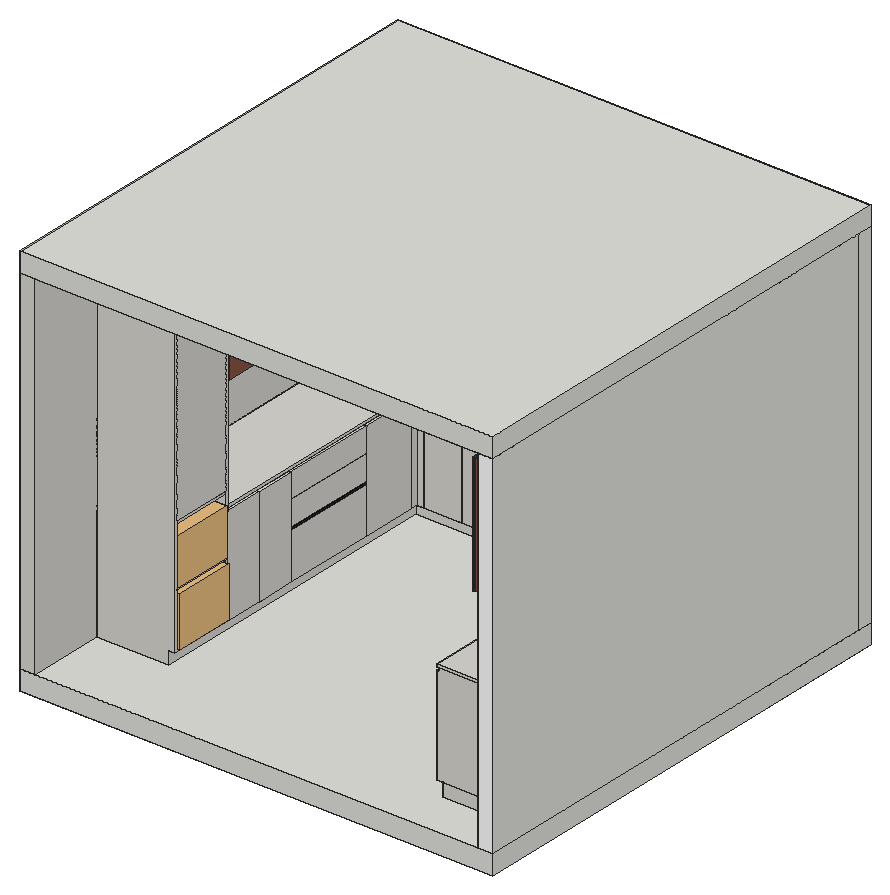
# SketchUp Ruby script. Lengths in inches.
U = 1.inch
M = Sketchup.active_model
def pt(a) = Geom::Point3d.new(a.map { |v| v * U })
def face(e, loops, mat)
  f = e.add_face(loops[0].map { |a| pt(a) })
  loops[1..].each { |l| e.add_face(l.map { |a| pt(a) }).erase! }
  f.material = f.back_material = mat if mat
  f
end
# faces: each face lists its corners as indices into pts; further lists are holes
def faces(e, pts, list, mat = nil) = list.each { |f| face(e, (f[0].is_a?(Array) ? f : [f]).map { |l| l.map { |i| pts[i] } }, mat) }
# xy, xz, yz: faces in a plane at the given z, y or x. An outline is a flat list of corners, or four numbers for a rectangle; further outlines are holes
def ring(l) = l.size == 4 ? [[l[0], l[1]], [l[2], l[1]], [l[2], l[3]], [l[0], l[3]]] : l.each_slice(2).to_a
def flat(e, list, mat, &to3) = list.each { |f| face(e, (f[0].is_a?(Array) ? f : [f]).map { |l| ring(l).map { |u, v| to3.(u, v) } }, mat) }
def xy(e, z, list, mat = nil) = flat(e, list, mat) { |x, y| [x, y, z] }
def xz(e, y, list, mat = nil) = flat(e, list, mat) { |x, z| [x, y, z] }
def yz(e, x, list, mat = nil) = flat(e, list, mat) { |y, z| [x, y, z] }
def lines(e, pts, list) = list.each { |a, b| e.add_line(pt(pts[a]), pt(pts[b])) }
# prism: a flat outline (further loops are holes) pulled along v
def prism(e, loops, v, mat = nil)
  f = face(e, loops, mat); d = Geom::Vector3d.new(v.map { |x| x * U })
  f.pushpull(f.normal.samedirection?(d) ? d.length : -d.length)
end
def box(e, o, s, mat = nil) = prism(e, [[o, [o[0] + s[0], o[1], o[2]], [o[0] + s[0], o[1] + s[1], o[2]], [o[0], o[1] + s[1], o[2]]]], [0, 0, s[2]], mat)
def at(x, y, z, deg = 0) = Geom::Transformation.translation(pt([x, y, z])) * Geom::Transformation.rotation(ORIGIN, Z_AXIS, deg.degrees)
def axes(o, x, y, z) = Geom::Transformation.new([*x, 0, *y, 0, *z, 0, *pt(o).to_a, 1])
def part(name) = M.definitions.add(name)
# library, detail: a bought-in or finely detailed component or shape, given as its bounding box
def library(name, o, s) = part(name).tap { |d| box(d.entities, o, s) }
def detail(e, o, s) = box(e.add_group.entities, o, s)
def put(e, d, t, mat = nil) = e.add_instance(d, t).tap { |i| i.material = mat if mat }
def group(e, t, mat = nil) = e.add_group.tap { |g| g.transformation = t; g.material = mat if mat }.entities
root = M.entities
M.materials.add("Pionite-a-Panolam-Brand-Canyon-Shadow-SO200-4K").color = [135, 86, 67]
M.materials.add("Tafisa-Cachemire-or-Cashmere-PM776-4K").color = [217, 215, 209]
M.materials.add("[Color M00]").color = [255, 255, 255]
M.materials.add("[Color M09]").color = [0, 0, 0]
M.materials.add("[Translucent Glass Gray]").color = [128, 128, 128]
M.materials["[Translucent Glass Gray]"].alpha = 0.5
c1 = library("Bowl 296 012 003",[-3.97,-3.98,-0.03],[7.96,7.96,3.84])
c2 = library("Cooker 143 035",[-7,-5.69,0],[14,11.41,9.46])
c3 = library("Cup 287 006 002",[-2.07,-2.07,-0.01],[4.14,4.15,3.07])
c4 = library("Kitchen Props 134 014",[-15.6875,-7.04,0],[31.37,14.09,12.97])
c5 = library("2-FOUR H60 CLC2",[0,-1.47,0],[23.5,21.86,23.5])
c6 = library("2-MICRO H40 CLC2",[0,-1.47,0],[23.5,21.86,15.63])
c7 = library("Stand 298 006",[-6.74,-6.74,-0.04],[13.48,13.48,13.7])
c8 = library("Bowl 298 014 002",[-6.91,-6.91,-0.04],[13.82,13.82,6.19])
c9 = library("Jug 155 004",[-2.86,-2.52,0],[7.11,5.04,4.97])
c10 = library("Jar 134 013",[-1.97,-1.98,0],[3.94,3.95,4.83])
c11 = library("Candle 160 011",[-1.94,-2,0],[3.88,3.94,4.57])
c12 = library("Jar 83-03",[-2.15,-2.09,0],[4.3,4.18,5.88])
c13 = library("5-HOTTE ASPIRANTE CLC2",[-15.16,-17.72,-0.29],[30.34,17.72,30.09])
c14 = library("Wicker-wood basket",[2.36,-2.2,-7.41],[20.73,22.5,7.78])
c15 = part("Group\#13")
box(c15.entities,[0,0,-0.71],[22.83,18.58,0.71])
c16 = library("Группа\#68",[0,0,-0.08],[23.6,20.47,1.99])
c17 = part("Group\#31")
xy(c17.entities,0,[[0.93,0,0.71,0.01,0.49,0.07,0.31,0.1875,0.16,0.35,0.05,0.54,0,0.76,0.01,0.98,0.07,1.1875,0.1875,1.375,0.35,1.53,0.54,1.63,0.76,1.68,0.98,1.68,1.1875,1.61,1.375,1.5,1.53,1.33,1.63,1.14,1.68,0.93,1.68,0.71,1.61,0.49,1.5,0.31,1.33,0.16,1.14,0.05]])
xz(root,126.85,[[20.33,66.28,37.04,101.29],[107.08,66.28,123.67,101.29]],"[Translucent Glass Gray]")
yz(root,17.15,[[107.09,66.28,123.67,101.29]],"[Translucent Glass Gray]")
yz(root,126.85,[[107.375,66.28,123.67,101.29]],"[Translucent Glass Gray]")
put(root,c1,at(32.52,133.57,66.28))
put(root,c1,at(24.37,133.35,66.28))
put(root,c2,at(33.29,126.21,41.57))
put(root,c3,at(32.73,133.83,78.66))
put(root,c3,at(28.04,133.83,78.66))
put(root,c3,at(23.35,133.83,78.66))
put(root,c4,axes([122.51,100.875,41.57],[-1,0,0],[0,1,0],[0,0,1]))
put(root,c5,axes([28.46,24.09,11.01],[0,0.79062,0],[-0.71131,0,0],[0,0,0.64648]))
put(root,c6,axes([28,24.09,27.71],[0,0.79062,0],[-0.6156,0,0],[0,0,0.91109]))
put(root,c7,axes([120.65,133.01,66.3],[0.3355,0,0],[0,0.3355,0],[0,0,0.3355]))
put(root,c7,axes([115.03,133.01,66.3],[0.3355,0,0],[0,0.3355,0],[0,0,0.3355]))
put(root,c7,axes([109.78,133.01,66.3],[0.3355,0,0],[0,0.3355,0],[0,0,0.3355]))
put(root,c8,axes([34.09,132.09,90.3],[0.31894,0,0],[0,0.31894,0],[0,0,0.31894]))
put(root,c8,axes([28.66,132.09,90.3],[0.31894,0,0],[0,0.31894,0],[0,0,0.31894]))
put(root,c8,axes([23.47,132.09,90.3],[0.31894,0,0],[0,0.31894,0],[0,0,0.31894]))
put(root,c9,axes([120.81,133.09,78.66],[0.59397,0.59397,0],[-0.59397,0.59397,0],[0,0,0.84]))
put(root,c9,axes([115.38,133.09,78.66],[0.59397,0.59397,0],[-0.59397,0.59397,0],[0,0,0.84]))
put(root,c9,axes([109.94,133.09,78.66],[0.59397,0.59397,0],[-0.59397,0.59397,0],[0,0,0.84]))
put(root,c10,at(120.52,132.59,90.33))
put(root,c11,axes([16.52,127.52,41.57],[1.7,0,0],[0,1.7,0],[0,0,1.7]))
put(root,c12,at(115,132.73,90.33))
put(root,c12,at(109.8,132.73,90.33))
put(root,c13,axes([72.24,139.5,63.27],[0.99919,0,0],[0,1,0],[0,0,1]))
g1 = group(root,at(0,0,0))
box(g1,[0,0,0],[144,144,6])
g2 = group(root,at(0,139.5,6))
xy(g2,0,[[0,0,144,4.5]])
xy(g2,108,[[0,0,144,4.5]])
xz(g2,0,[[[0,0,144,108],[4.5,35.57,139.5,59.57]],[4.5,35.57,139.5,59.57]])
xz(g2,4.5,[[0,0,144,108]])
yz(g2,0,[[0,0,4.5,108]])
yz(g2,144,[[0,0,4.5,108]])
g3 = group(root,at(139.5,0,6))
xy(g3,0,[[0,0,4.5,139.5]])
xy(g3,108,[[0,0,4.5,139.5]],"[Color M00]")
xz(g3,0,[[0,0,4.5,108]],"[Color M00]")
xz(g3,139.5,[[0,0,4.5,108]])
yz(g3,0,[[0,0,0,108,139.5,108,139.5,59.57,14.26,59.57,14.26,35.57,139.5,35.57,139.5,0],[14.26,35.57,139.5,59.57]])
yz(g3,4.5,[[0,0,139.5,108]])
g4 = group(root,at(0,0,6),"Tafisa-Cachemire-or-Cashmere-PM776-4K")
xy(g4,0,[[0,0,4.5,139.5]])
xy(g4,108,[[0,0,4.5,139.5]])
xz(g4,0,[[0,0,4.5,108]])
xz(g4,139.5,[[0,0,4.5,108]])
yz(g4,0,[[0,0,139.5,108]])
yz(g4,4.5,[[0,0,139.5,0,139.5,35.57,43.38,35.57,43.38,59.57,139.5,59.57,139.5,108,0,108],[43.38,35.57,139.5,59.57]])
g5 = group(root,at(4.5,0,6),"Tafisa-Cachemire-or-Cashmere-PM776-4K")
xy(g5,0,[[113,14.26,113,117.5,22,117.5,22,23.38,0,23.38,0,139.5,135,139.5,135,14.26]])
xy(g5,4,[[111,14.26,111,38.26,111.71,38.26,111.71,38.38,111,38.38,111,50.26,111.71,50.26,111.71,50.38,111,50.38,111,62.26,111.71,62.26,111.71,62.38,111,62.38,111,72.38,111.71,72.38,111.71,72.5,111,72.5,111,99.38,111.71,99.38,111.71,99.5,111,99.5,111,113.38,111.71,113.38,111.71,113.5,111,113.5,111,115.5,113,115.5,113,14.26],[22,23.38,22,115.5,24,115.5,24,113.5,23.29,113.5,23.29,113.38,24,113.38,24,96.5,23.29,96.5,23.29,96.38,24,96.38,24,67.62,23.29,67.62,23.29,67.5,24,67.5,24,55.5,23.29,55.5,23.29,55.38,24,55.38,24,43.5,23.29,43.5,23.29,43.38,24,43.38,24,23.38],[22,115.5,22,117.5,113,117.5,113,115.5,109.12,115.5,109.12,116.21,109,116.21,109,115.5,97.37,115.5,97.37,116.21,97.25,116.21,97.25,115.5,85.5,115.5,85.5,116.21,85.38,116.21,85.38,115.5,49.62,115.5,49.62,116.21,26,116.21,26,115.5],[26.12,115.5,37.75,116.21],[37.87,115.5,49.5,116.21]])
xy(g5,4.71,[[111,14.97,133.83,37.56],[1.17,24.09,24,42.67]])
xy(g5,18.02,[[111,72.5,111.71,99.38]])
xy(g5,18.02,[[23.29,67.62,24,96.38],[49.62,115.5,85.38,116.21]],"[Color M09]")
xy(g5,19,[[111,72.5,111.71,99.38]])
xy(g5,19,[[23.29,67.62,24,96.38],[49.62,115.5,85.38,116.21]],"[Color M09]")
xy(g5,26.5,[[23.29,67.62,24,96.38],[111,72.5,111.71,99.38],[49.62,115.5,85.38,116.21]])
xy(g5,26.62,[[23.29,67.62,24,96.38],[111,72.5,111.71,99.38],[49.62,115.5,85.38,116.21]])
xy(g5,33.29,[[111,14.97,133.83,37.56]])
xy(g5,34,[[111,14.26,111.71,38.26],[111,38.38,111.71,50.26],[23.29,43.5,24,55.38],[111,50.38,111.71,62.26],[23.29,55.5,24,67.5],
  [111,62.38,111.71,72.38],[23.29,67.62,24,96.38],[111,72.5,111.71,99.38],[23.29,96.5,24,113.38],[111,99.5,111.71,113.38],
  [23.29,113.5,24,115.5],[111,113.5,111.71,115.5],[23.29,115.5,26,116.21],[26.12,115.5,37.75,116.21],[37.87,115.5,49.5,116.21],
  [49.62,115.5,85.38,116.21],[85.5,115.5,97.25,116.21],[97.37,115.5,109,116.21],[109.12,115.5,111.71,116.21]])
xy(g5,34.79,[[111,14.26,111.71,115.5],[23.29,43.5,24,115.5],[23.29,115.5,111.71,116.21]])
xy(g5,35.57,[[111,14.26,135,14.26,135,139.5,0,139.5,0,43.38,23.29,43.38,23.29,43.5,24,43.5,24,115.5,111,115.5]])
xy(g5,39.83,[[1.17,24.09,1.17,42.67,23.29,42.67,23.29,42.56,24,42.56,24,24.21,23.29,24.21,23.29,24.09]])
xy(g5,107.17,[[23.29,24.21,24,42.56]])
xy(g5,107.29,[[1.17,24.09,23.29,42.67],[23.29,24.09,24,24.21],[23.29,24.21,24,42.56],[23.29,42.56,24,42.67]])
xy(g5,108,[[0,23.38,24,43.38]])
xz(g5,14.26,[[113,0,135,4],[111,4,135,4,135,34.79,111.71,34.79,111.71,34,111,34],[111,34.79,135,35.57]])
xz(g5,14.97,[[111,4.71,133.83,33.29]])
xz(g5,23.38,[[0,0,22,0,22,4,24,4,24,108,0,108]])
xz(g5,24.09,[[1.17,4.71,24,39.83],[1.17,39.83,23.29,107.29],[23.29,39.83,24,107.29]])
xz(g5,24.21,[[23.29,39.83,24,107.17]])
xz(g5,37.56,[[111,4.71,133.83,33.29]])
xz(g5,38.26,[[111,4,111.71,34]])
xz(g5,38.38,[[111,4,111.71,34]])
xz(g5,42.56,[[23.29,39.83,24,107.17]])
xz(g5,42.67,[[1.17,4.71,24,39.83],[1.17,39.83,23.29,107.29],[23.29,39.83,24,107.29]])
xz(g5,43.38,[[23.29,4,24,34],[23.29,34,24,34.79],[23.29,34.79,24,108],[0,35.57,23.29,108]])
xz(g5,43.5,[[23.29,4,24,34],[23.29,34.79,24,35.57]])
xz(g5,50.26,[[111,4,111.71,34]])
xz(g5,50.38,[[111,4,111.71,34]])
xz(g5,55.38,[[23.29,4,24,34]])
xz(g5,55.5,[[23.29,4,24,34]])
xz(g5,62.26,[[111,4,111.71,34]])
xz(g5,62.38,[[111,4,111.71,34]])
xz(g5,67.5,[[23.29,4,24,18.02],[23.29,18.02,24,19],[23.29,19,24,26.5],[23.29,26.5,24,26.62],[23.29,26.62,24,34]])
xz(g5,67.62,[[23.29,4,24,18.02],[23.29,19,24,26.5],[23.29,26.62,24,34]])
xz(g5,72.38,[[111,4,111.71,18.02],[111,18.02,111.71,19],[111,19,111.71,26.5],[111,26.5,111.71,26.62],[111,26.62,111.71,34]])
xz(g5,72.5,[[111,4,111.71,18.02],[111,19,111.71,26.5],[111,26.62,111.71,34]])
xz(g5,96.38,[[23.29,4,24,18.02],[23.29,19,24,26.5],[23.29,26.62,24,34]])
xz(g5,96.5,[[23.29,4,24,18.02],[23.29,18.02,24,19],[23.29,19,24,26.5],[23.29,26.5,24,26.62],[23.29,26.62,24,34]])
xz(g5,99.38,[[111,4,111.71,18.02],[111,19,111.71,26.5],[111,26.62,111.71,34]])
xz(g5,99.5,[[111,4,111.71,34]])
xz(g5,113.38,[[23.29,4,24,34],[111,4,111.71,34]])
xz(g5,113.5,[[23.29,4,24,34],[111,4,111.71,34]])
xz(g5,115.5,[[24,4,26,34],[26.12,4,37.75,34],[37.87,4,49.5,34],[49.62,4,85.38,18.02],[85.5,4,97.25,34],
  [97.37,4,109,34],[109.12,4,111,34],[49.62,19,85.38,26.5],[49.62,26.62,85.38,34],[24,34.79,111,35.57]])
xz(g5,116.21,[[26,4,26.12,34],[26.12,4,37.75,34],[37.75,4,37.87,34],[37.87,4,49.5,34],[49.5,4,49.62,18.02],
  [85.38,4,85.5,18.02],[97.25,4,97.37,34],[109,4,109.12,34],[49.5,19,49.62,26.5],[85.38,19,85.5,26.5],
  [49.5,26.5,85.5,26.62],[49.5,26.62,49.62,34],[85.38,26.62,85.5,34]])
xz(g5,116.21,[[49.5,18.02,85.5,19],[23.29,34,111.71,34.79]],"[Color M09]")
xz(g5,117.5,[[22,0,113,4]])
xz(g5,139.5,[[0,0,135,34],[0,34,135,34.79],[0,34.79,135,35.57]])
yz(g5,0,[[23.38,0,139.5,34],[23.38,34,139.5,34.79],[23.38,34.79,23.38,108,43.38,108,43.38,35.57,139.5,35.57,139.5,34.79]])
yz(g5,1.17,[[24.09,4.71,42.67,39.83],[24.09,39.83,42.67,107.29]])
yz(g5,22,[[23.38,0,117.5,4]])
yz(g5,23.29,[[43.38,4,43.5,34],[55.38,4,55.5,34],[67.5,4,67.62,18.02],[96.38,4,96.5,18.02],[113.38,4,113.5,34],
  [67.5,19,67.62,26.5],[96.38,19,96.5,26.5],[67.5,26.5,96.5,26.62],[67.5,26.62,67.62,34],[96.38,26.62,96.5,34],
  [43.38,34.79,43.5,35.57],[24.09,39.83,24.21,107.29],[42.56,39.83,42.67,107.29],[24.21,107.17,42.56,107.29]])
yz(g5,23.29,[[67.5,18.02,96.5,19],[43.38,34,116.21,34.79]],"[Color M09]")
yz(g5,24,[[[23.38,4,43.38,108],[24.09,4.71,42.67,107.29]],[43.5,4,55.38,34],[55.5,4,67.5,34],[67.62,4,96.38,18.02],[96.5,4,113.38,34],
  [113.5,4,115.5,34],[67.62,19,96.38,26.5],[67.62,26.62,96.38,34],[43.5,34.79,115.5,35.57],[24.21,39.83,42.56,107.17]])
yz(g5,26,[[115.5,4,116.21,34]])
yz(g5,26.12,[[115.5,4,116.21,34]])
yz(g5,37.75,[[115.5,4,116.21,34]])
yz(g5,37.87,[[115.5,4,116.21,34]])
yz(g5,49.5,[[115.5,4,116.21,18.02],[115.5,18.02,116.21,19],[115.5,19,116.21,26.5],[115.5,26.5,116.21,26.62],[115.5,26.62,116.21,34]])
yz(g5,49.62,[[115.5,4,116.21,18.02],[115.5,19,116.21,26.5],[115.5,26.62,116.21,34]])
yz(g5,85.38,[[115.5,4,116.21,18.02],[115.5,19,116.21,26.5],[115.5,26.62,116.21,34]])
yz(g5,85.5,[[115.5,4,116.21,18.02],[115.5,18.02,116.21,19],[115.5,19,116.21,26.5],[115.5,26.5,116.21,26.62],[115.5,26.62,116.21,34]])
yz(g5,97.25,[[115.5,4,116.21,34]])
yz(g5,97.37,[[115.5,4,116.21,34]])
yz(g5,109,[[115.5,4,116.21,34]])
yz(g5,109.12,[[115.5,4,116.21,34]])
yz(g5,111,[[[14.26,4,38.26,34],[14.97,4.71,37.56,33.29]],[38.38,4,50.26,34],[50.38,4,62.26,34],[62.38,4,72.38,34],[72.5,4,99.38,18.02],
  [99.5,4,113.38,34],[113.5,4,115.5,34],[72.5,19,99.38,26.5],[72.5,26.62,99.38,34],[14.26,34.79,115.5,35.57]])
yz(g5,111.71,[[38.26,4,38.38,34],[50.26,4,50.38,34],[62.26,4,62.38,34],[72.38,4,72.5,18.02],[99.38,4,99.5,34],
  [113.38,4,113.5,34],[72.38,19,72.5,26.5],[72.38,26.5,99.38,26.62],[72.38,26.62,72.5,34]])
yz(g5,111.71,[[72.38,18.02,99.38,19],[14.26,34,116.21,34.79]],"[Color M09]")
yz(g5,113,[[14.26,0,117.5,4]])
yz(g5,133.83,[[14.97,4.71,37.56,33.29]])
yz(g5,135,[[14.26,0,139.5,34],[14.26,34,139.5,34.79],[14.26,34.79,139.5,35.57]])
put(g5,c14,at(109,17.26,12.81))
put(g5,c14,at(109,17.26,22.11))
put(g5,c14,at(108.64,17.26,31.4))
put(g5,c15,at(1.17,24.09,21.71))
put(g5,c15,at(1.17,24.09,39.71))
g6 = group(root,at(4.5,43.38,65.57),"Pionite-a-Panolam-Brand-Canyon-Shadow-SO200-4K")
xy(g6,0,[[122.71,-29.12,122.71,81.12,122,81.12,122,83.12,120,83.12,120,83.83,15,83.83,15,83.12,13,83.12,13,81.12,12.29,81.12,12.29,0,0,0,0,96.12,135,96.12,135,-29.12],[122,-29.12,122.71,-7.83],[122,-7.72,122.71,10.17],[12.29,0,13,14.38],[122,10.28,122.71,28.17],
  [12.29,14.5,13,28.88],[122,28.28,122.71,46.17],[12.29,29,13,45.88],[12.29,46,13,62.88],[122,46.28,122.71,63.17],
  [122,63.28,122.71,81],[33.37,83.12,51.5,83.83],[51.62,83.12,67.5,83.83],[67.62,83.12,83.5,83.83],[83.62,83.12,101.75,83.83]])
xy(g6,0,[[12.29,63,13,81],[15.12,83.12,33.25,83.83],[101.87,83.12,119.88,83.83]],"[Color M09]")
xy(g6,0.71,[[1,63.71,12.29,80.29],[122.71,63.99,134,80.29],[15.83,83.83,32.54,95.12],[102.58,83.83,119.17,95.12]])
xy(g6,0.71,[[12.29,63.71,13,80.29],[122,63.99,122.71,80.29],[15.83,83.12,32.54,83.83],[102.58,83.12,119.17,83.83]],"[Color M09]")
xy(g6,35.72,[[1,63.71,12.29,80.29],[122.71,63.99,134,80.29],[15.83,83.83,32.54,95.12],[102.58,83.83,119.17,95.12]])
xy(g6,35.72,[[12.29,63.71,13,80.29],[122,63.99,122.71,80.29],[15.83,83.12,32.54,83.83],[102.58,83.12,119.17,83.83]],"[Color M09]")
xy(g6,36.43,[[122.71,-29.12,135,-29.12,135,96.12,0,96.12,0,0,12.29,0,12.29,81.12,13,81.12,13,83.12,15,83.12,15,83.83,120,83.83,120,83.12,122,83.12,122,81.12,122.71,81.12],[122,-29.12,122.71,-7.83],[122,-7.72,122.71,10.17],[12.29,0,13,14.38],[122,10.28,122.71,28.17],
  [12.29,14.5,13,28.88],[122,28.28,122.71,46.17],[12.29,29,13,45.88],[12.29,46,13,62.88],[122,46.28,122.71,63.17],
  [33.37,83.12,51.5,83.83],[51.62,83.12,67.5,83.83],[67.62,83.12,83.5,83.83],[83.62,83.12,101.75,83.83]])
xy(g6,36.43,[[12.29,63,13,81],[122,63.28,122.71,81],[15.12,83.12,33.25,83.83],[101.87,83.12,119.88,83.83]],"[Color M09]")
xz(g6,-29.12,[[122,0,122.71,36.43],[122.71,0,135,36.43]])
xz(g6,-7.83,[[122,0,122.71,36.43]])
xz(g6,-7.72,[[122,0,122.71,36.43]])
xz(g6,0,[[0,0,12.29,36.43],[12.29,0,13,36.43]])
xz(g6,10.17,[[122,0,122.71,36.43]])
xz(g6,10.28,[[122,0,122.71,36.43]])
xz(g6,14.38,[[12.29,0,13,36.43]])
xz(g6,14.5,[[12.29,0,13,36.43]])
xz(g6,28.17,[[122,0,122.71,36.43]])
xz(g6,28.28,[[122,0,122.71,36.43]])
xz(g6,28.88,[[12.29,0,13,36.43]])
xz(g6,29,[[12.29,0,13,36.43]])
xz(g6,45.88,[[12.29,0,13,36.43]])
xz(g6,46,[[12.29,0,13,36.43]])
xz(g6,46.17,[[122,0,122.71,36.43]])
xz(g6,46.28,[[122,0,122.71,36.43]])
xz(g6,62.88,[[12.29,0,13,36.43]])
xz(g6,63,[[12.29,0,13,36.43]],"[Color M09]")
xz(g6,63.17,[[122,0,122.71,36.43]])
xz(g6,63.28,[[122,0,122.71,36.43]],"[Color M09]")
xz(g6,63.71,[[1,0.71,12.29,12.38],[12.29,0.71,13,35.72],[1,12.38,12.29,35.72]])
xz(g6,63.99,[[122,0.71,122.71,35.72],[122.71,0.71,134,12.38],[122.71,12.38,134,35.72]])
xz(g6,80.29,[[1,0.71,12.29,35.72],[122.71,0.71,134,12.38],[122.71,12.38,134,35.72]])
xz(g6,80.29,[[12.29,0.71,13,35.72],[122,0.71,122.71,35.72]],"[Color M09]")
xz(g6,81,[[122,0,122.71,36.43]])
xz(g6,81,[[12.29,0,13,36.43]],"[Color M09]")
xz(g6,81.12,[[12.29,0,13,36.43],[122,0,122.71,36.43]])
xz(g6,83.12,[[13,0,15,36.43],[33.37,0,51.5,36.43],[51.62,0,67.5,36.43],[67.62,0,83.5,36.43],[83.62,0,101.75,36.43],
  [120,0,122,36.43]])
xz(g6,83.12,[[[15.12,0,33.25,36.43],[15.83,0.71,32.54,35.72]],[[101.87,0,119.88,36.43],[102.58,0.71,119.17,35.72]]],"[Color M09]")
xz(g6,83.83,[[15,0,15.12,36.43],[[15.12,0,33.25,36.43],[15.83,0.71,32.54,35.72]],[33.25,0,33.37,36.43],[33.37,0,51.5,36.43],[51.5,0,51.62,36.43],
  [51.62,0,67.5,36.43],[67.5,0,67.62,36.43],[67.62,0,83.5,36.43],[83.5,0,83.62,36.43],[83.62,0,101.75,36.43],
  [101.75,0,101.87,36.43],[[101.87,0,119.88,36.43],[102.58,0.71,119.17,35.72]],[119.88,0,120,36.43]])
xz(g6,95.12,[[15.83,0.71,32.54,12.38],[102.58,0.71,119.17,12.38],[15.83,12.38,32.54,35.72],[102.58,12.38,119.17,35.72]])
xz(g6,96.12,[[0,0,135,36.43]])
yz(g6,0,[[0,0,96.12,36.43]])
yz(g6,1,[[63.71,0.71,80.29,12.38],[63.71,12.38,80.29,35.72]])
yz(g6,12.29,[[0,0,14.38,36.43],[14.38,0,14.5,36.43],[14.5,0,28.88,36.43],[28.88,0,29,36.43],[29,0,45.88,36.43],
  [45.88,0,46,36.43],[46,0,62.88,36.43],[62.88,0,63,36.43],[[63,0,81,36.43],[63.71,0.71,80.29,35.72]],[81,0,81.12,36.43]])
yz(g6,13,[[0,0,14.38,36.43],[14.5,0,28.88,36.43],[29,0,45.88,36.43],[46,0,62.88,36.43],[81.12,0,83.12,36.43]])
yz(g6,13,[[[63,0,81,36.43],[63.71,0.71,80.29,35.72]]],"[Color M09]")
yz(g6,15,[[83.12,0,83.83,36.43]])
yz(g6,15.12,[[83.12,0,83.83,36.43]],"[Color M09]")
yz(g6,15.83,[[83.83,0.71,95.12,12.38],[83.83,12.38,95.12,35.72]])
yz(g6,15.83,[[83.12,0.71,83.83,35.72]],"[Color M09]")
yz(g6,32.54,[[83.83,0.71,95.12,12.38],[83.83,12.38,95.12,35.72]])
yz(g6,32.54,[[83.12,0.71,83.83,35.72]],"[Color M09]")
yz(g6,33.25,[[83.12,0,83.83,36.43]],"[Color M09]")
yz(g6,33.37,[[83.12,0,83.83,36.43]])
yz(g6,51.5,[[83.12,0,83.83,36.43]])
yz(g6,51.62,[[83.12,0,83.83,36.43]])
yz(g6,67.5,[[83.12,0,83.83,36.43]])
yz(g6,67.62,[[83.12,0,83.83,36.43]])
yz(g6,83.5,[[83.12,0,83.83,36.43]])
yz(g6,83.62,[[83.12,0,83.83,36.43]])
yz(g6,101.75,[[83.12,0,83.83,36.43]])
yz(g6,101.87,[[83.12,0,83.83,36.43]],"[Color M09]")
yz(g6,102.58,[[83.83,0.71,95.12,12.38],[83.83,12.38,95.12,35.72]])
yz(g6,102.58,[[83.12,0.71,83.83,35.72]],"[Color M09]")
yz(g6,119.17,[[83.83,0.71,95.12,12.38],[83.83,12.38,95.12,35.72]])
yz(g6,119.17,[[83.12,0.71,83.83,35.72]],"[Color M09]")
yz(g6,119.88,[[83.12,0,83.83,36.43]],"[Color M09]")
yz(g6,120,[[83.12,0,83.83,36.43]])
yz(g6,122,[[-29.12,0,-7.83,36.43],[-7.72,0,10.17,36.43],[10.28,0,28.17,36.43],[28.28,0,46.17,36.43],[46.28,0,63.17,36.43],
  [81.12,0,83.12,36.43]])
yz(g6,122,[[[63.28,0,81,36.43],[63.99,0.71,80.29,35.72]]],"[Color M09]")
yz(g6,122.71,[[-29.12,0,-7.83,36.43],[-7.83,0,-7.72,36.43],[-7.72,0,10.17,36.43],[10.17,0,10.28,36.43],[10.28,0,28.17,36.43],
  [28.17,0,28.28,36.43],[28.28,0,46.17,36.43],[46.17,0,46.28,36.43],[46.28,0,63.17,36.43],[63.17,0,63.28,36.43],
  [[63.28,0,81,36.43],[63.99,0.71,80.29,35.72]],[81,0,81.12,36.43]])
yz(g6,134,[[63.99,0.71,80.29,12.38],[63.99,12.38,80.29,35.72]])
yz(g6,135,[[-29.12,0,96.12,36.43]])
g7 = group(g6,at(15.83,83.83,12.38))
box(g7,[0,1,0],[16.71,10.29,0.71])
g8 = group(g6,at(15.83,83.83,24.05))
box(g8,[0,1,0],[16.71,10.29,0.71])
g9 = group(g6,at(102.58,83.83,12.38))
box(g9,[0,1,0],[16.6,10.29,0.71])
g10 = group(g6,at(102.58,83.83,24.05))
box(g10,[0,1,0],[16.6,10.29,0.71])
g11 = group(g6,at(122.71,63.99,12.38))
box(g11,[0,0,-0.71],[11.29,16.3,0.71])
g12 = group(g6,at(122.71,63.99,24.05))
box(g12,[0,0,-0.71],[11.29,16.3,0.71])
g13 = group(g6,at(1,63.71,12.38))
box(g13,[0,0,-0.71],[11.29,16.58,0.71])
g14 = group(g6,at(1,63.71,24.05))
box(g14,[0,0,-0.71],[11.29,16.58,0.71])
put(root,c16,axes([56.19,116.41,42.28],[1.4136,0,0],[0,1,0],[0,0,1]))
g15 = group(root,at(0,0,114))
xy(g15,0,[[[0,0,144,144],[36.07,29.1,107.32,107.47]],[36.07,29.1,36.07,56.28,36.85,56.28,36.85,29.88,59.69,29.88,59.69,29.1],[36.85,29.88,106.53,106.68],[106.53,80.28,106.53,106.68,83.69,106.68,83.69,107.47,107.32,107.47,107.32,80.28]])
xy(g15,6,[[0,0,144,144]])
xz(g15,0,[[0,0,144,6]])
xz(g15,144,[[0,0,144,6]])
yz(g15,0,[[0,0,144,6]])
yz(g15,144,[[0,0,144,6]])
g16 = group(g15,at(36.07,56.28,0))
xy(g16,0,[[0,0,0,51.1875,47.625,51.1875,47.625,50.4,0.79,50.4,0.79,0]])
g17 = group(g15,at(59.69,29.1,0))
xy(g17,0,[[0,0,0,0.79,46.84,0.79,46.84,51.1875,47.625,51.1875,47.625,0]])
g18 = group(root,at(30.95,109.95,114))
detail(g18,[0,0,-0.24],[3.11,3.11,0.24])
put(g18,c17,at(0.71,0.71,-0.11))
g19 = group(root,at(110.24,109.95,114))
detail(g19,[0,0,-0.24],[3.11,3.11,0.24])
put(g19,c17,at(0.71,0.71,-0.11))
g20 = group(root,at(86.24,109.95,114))
detail(g20,[0,0,-0.24],[3.11,3.11,0.24])
put(g20,c17,at(0.71,0.71,-0.11))
g21 = group(root,at(58.49,109.95,114))
detail(g21,[0,0,-0.24],[3.11,3.11,0.24])
put(g21,c17,at(0.71,0.71,-0.11))
g22 = group(root,at(30.95,85.95,114))
detail(g22,[0,0,-0.24],[3.11,3.11,0.24])
put(g22,c17,at(0.71,0.71,-0.11))
g23 = group(root,at(30.95,61.95,114))
detail(g23,[0,0,-0.24],[3.11,3.11,0.24])
put(g23,c17,at(0.71,0.71,-0.11))
g24 = group(root,at(110.24,85.95,114))
detail(g24,[0,0,-0.24],[3.11,3.11,0.24])
put(g24,c17,at(0.71,0.71,-0.11))
g25 = group(root,at(110.24,61.95,114))
detail(g25,[0,0,-0.24],[3.11,3.11,0.24])
put(g25,c17,at(0.71,0.71,-0.11))
g26 = group(root,at(110.24,37.95,114))
detail(g26,[0,0,-0.24],[3.11,3.11,0.24])
put(g26,c17,at(0.71,0.71,-0.11))
g27 = group(root,at(110.24,13.95,114))
detail(g27,[0,0,-0.24],[3.11,3.11,0.24])
put(g27,c17,at(0.71,0.71,-0.11))
g28 = group(root,at(86.24,18.26,114))
detail(g28,[0,0,-0.24],[3.11,3.11,0.24])
put(g28,c17,at(0.71,0.71,-0.11))
g29 = group(root,at(58.49,18.26,114))
detail(g29,[0,0,-0.24],[3.11,3.11,0.24])
put(g29,c17,at(0.71,0.71,-0.11))
g30 = group(root,at(30.95,47.2,114))
detail(g30,[0,0,-0.24],[3.11,3.11,0.24])
put(g30,c17,at(0.71,0.71,-0.11))
g31 = group(root,at(46.26,13.95,114))
detail(g31,[0,0,-0.24],[3.11,3.11,0.24])
put(g31,c17,at(0.71,0.71,-0.11))
